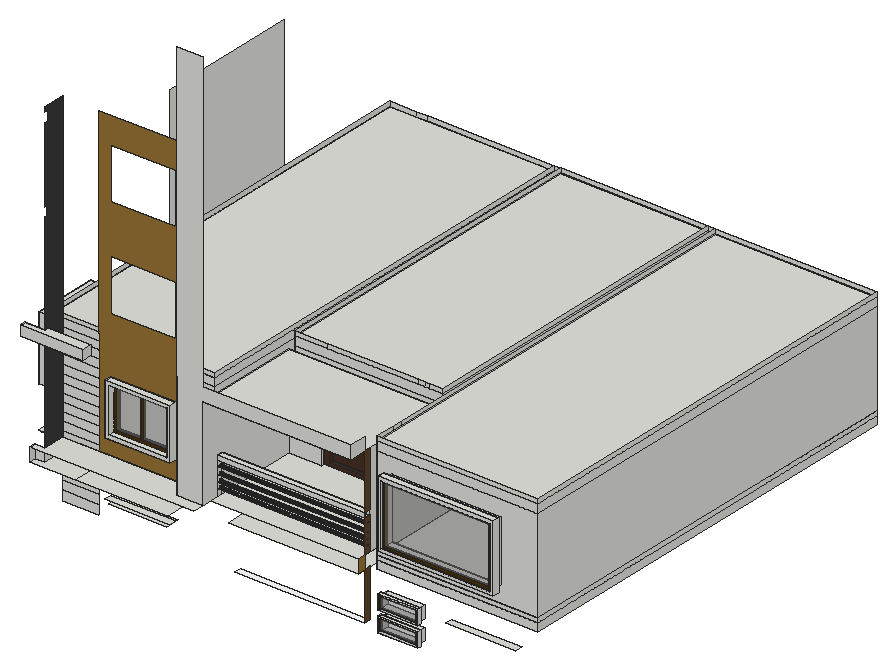
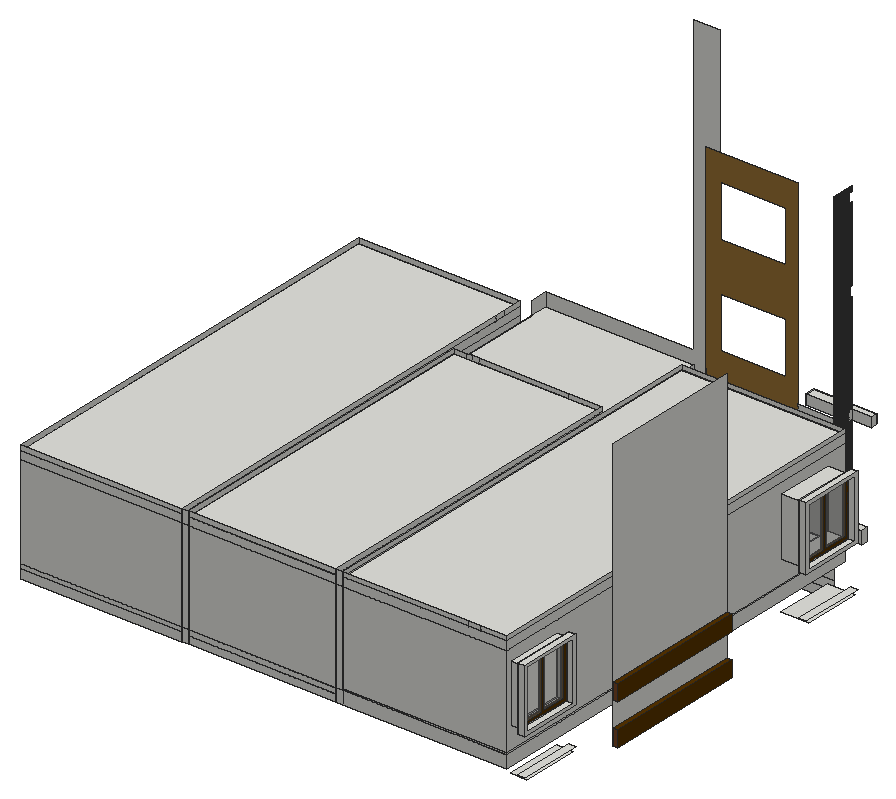
# SketchUp Ruby script. Lengths in inches.
U = 1.inch
M = Sketchup.active_model
def pt(a) = Geom::Point3d.new(a.map { |v| v * U })
def face(e, loops, mat)
  f = e.add_face(loops[0].map { |a| pt(a) })
  loops[1..].each { |l| e.add_face(l.map { |a| pt(a) }).erase! }
  f.material = f.back_material = mat if mat
  f
end
# faces: each face lists its corners as indices into pts; further lists are holes
def faces(e, pts, list, mat = nil) = list.each { |f| face(e, (f[0].is_a?(Array) ? f : [f]).map { |l| l.map { |i| pts[i] } }, mat) }
# xy, xz, yz: faces in a plane at the given z, y or x. An outline is a flat list of corners, or four numbers for a rectangle; further outlines are holes
def ring(l) = l.size == 4 ? [[l[0], l[1]], [l[2], l[1]], [l[2], l[3]], [l[0], l[3]]] : l.each_slice(2).to_a
def flat(e, list, mat, &to3) = list.each { |f| face(e, (f[0].is_a?(Array) ? f : [f]).map { |l| ring(l).map { |u, v| to3.(u, v) } }, mat) }
def xy(e, z, list, mat = nil) = flat(e, list, mat) { |x, y| [x, y, z] }
def xz(e, y, list, mat = nil) = flat(e, list, mat) { |x, z| [x, y, z] }
def yz(e, x, list, mat = nil) = flat(e, list, mat) { |y, z| [x, y, z] }
def lines(e, pts, list) = list.each { |a, b| e.add_line(pt(pts[a]), pt(pts[b])) }
# prism: a flat outline (further loops are holes) pulled along v
def prism(e, loops, v, mat = nil)
  f = face(e, loops, mat); d = Geom::Vector3d.new(v.map { |x| x * U })
  f.pushpull(f.normal.samedirection?(d) ? d.length : -d.length)
end
def box(e, o, s, mat = nil) = prism(e, [[o, [o[0] + s[0], o[1], o[2]], [o[0] + s[0], o[1] + s[1], o[2]], [o[0], o[1] + s[1], o[2]]]], [0, 0, s[2]], mat)
def at(x, y, z, deg = 0) = Geom::Transformation.translation(pt([x, y, z])) * Geom::Transformation.rotation(ORIGIN, Z_AXIS, deg.degrees)
def axes(o, x, y, z) = Geom::Transformation.new([*x, 0, *y, 0, *z, 0, *pt(o).to_a, 1])
def part(name) = M.definitions.add(name)
# library, detail: a bought-in or finely detailed component or shape, given as its bounding box
def library(name, o, s) = part(name).tap { |d| box(d.entities, o, s) }
def detail(e, o, s) = box(e.add_group.entities, o, s)
def put(e, d, t, mat = nil) = e.add_instance(d, t).tap { |i| i.material = mat if mat }
def group(e, t, mat = nil) = e.add_group.tap { |g| g.transformation = t; g.material = mat if mat }.entities
root = M.entities
M.materials.add("[Color C08]").color = [85, 51, 0]
M.materials.add("[Color D07]").color = [153, 114, 54]
M.materials.add("[Color D08]").color = [95, 67, 39]
M.materials.add("[Color M00]").color = [255, 255, 255]
M.materials.add("[Color M07]").color = [58, 58, 58]
M.materials.add("[Translucent Glass Gray]").color = [128, 128, 128]
M.materials["[Translucent Glass Gray]"].alpha = 0.5
M.materials.add("[Wood Veneer 01]").color = [71, 47, 37]
M.materials.add("[Wood Veneer 01]1").color = [120, 70, 37]
c1 = part("Group\#3")
xy(c1.entities,0,[[0,0,69.125,3.25]],"[Color C08]")
xy(c1.entities,1.72,[[1.72,0,67.41,3.25]],"[Color C08]")
xy(c1.entities,48.28,[[1.72,0,67.41,3.25]],"[Color C08]")
xy(c1.entities,50,[[0,0,69.125,3.25]],"[Color C08]")
xz(c1.entities,0,[[[0,0,69.125,50],[1.72,1.72,67.41,48.28]]],"[Color C08]")
xz(c1.entities,0,[[1.72,1.72,67.41,48.28]],"[Translucent Glass Gray]")
xz(c1.entities,3.25,[[[0,0,69.125,50],[1.72,1.72,67.41,48.28]]],"[Color C08]")
yz(c1.entities,0,[[0,0,3.25,50]],"[Color C08]")
yz(c1.entities,1.72,[[0,1.72,3.25,48.28]],"[Color C08]")
yz(c1.entities,67.41,[[0,1.72,3.25,48.28]],"[Color C08]")
yz(c1.entities,69.125,[[0,0,3.25,50]],"[Color C08]")
c2 = part("Group\#2")
xy(c2.entities,0,[[0,0,105.3125,8.625]],"[Wood Veneer 01]")
xy(c2.entities,6.5,[[6.5,0,98.81,8.625]],"[Wood Veneer 01]")
xy(c2.entities,132.37,[[6.5,0,98.81,8.625]],"[Wood Veneer 01]")
xy(c2.entities,138.875,[[0,0,105.3125,8.625]],"[Wood Veneer 01]")
xz(c2.entities,0,[[[0,0,105.3125,138.875],[6.5,6.5,98.81,132.37]]],"[Wood Veneer 01]")
xz(c2.entities,8.625,[[[0,0,105.3125,138.875],[6.5,6.5,98.81,132.37]],[6.5,6.5,98.81,132.37]],"[Wood Veneer 01]")
yz(c2.entities,0,[[0,0,8.625,138.875]],"[Wood Veneer 01]")
yz(c2.entities,6.5,[[0,6.5,8.625,132.37]],"[Wood Veneer 01]")
yz(c2.entities,98.81,[[0,6.5,8.625,132.37]],"[Wood Veneer 01]")
yz(c2.entities,105.3125,[[0,0,8.625,138.875]],"[Wood Veneer 01]")
c3 = part("Group\#4")
xy(c3.entities,0,[[0,0,0.4375,8.25]],"[Color C08]")
xy(c3.entities,9.875,[[0,0,0.4375,8.25]],"[Color C08]")
xz(c3.entities,0,[[0,0,0.4375,9.875]],"[Color C08]")
xz(c3.entities,0.45,[[0,0.45,0.4375,9.42]],"[Color C08]")
xz(c3.entities,4.05,[[0,0.49,0.4375,9.45]],"[Color C08]")
xz(c3.entities,4.38,[[0,0.49,0.4375,9.45]],"[Color C08]")
xz(c3.entities,7.8,[[0,0.45,0.4375,9.42]],"[Color C08]")
xz(c3.entities,8.25,[[0,0,0.4375,9.875]],"[Color C08]")
yz(c3.entities,0,[[[0,0,8.25,9.875],[0.45,0.45,4.05,0.49,4.05,9.45,0.45,9.42],[7.8,0.45,7.8,9.42,4.38,9.45,4.38,0.49]]],"[Color C08]")
yz(c3.entities,0,[[0.45,0.45,0.45,9.42,4.05,9.45,4.05,0.49],[7.8,0.45,4.38,0.49,4.38,9.45,7.8,9.42]],"[Translucent Glass Gray]")
yz(c3.entities,0.4375,[[[0,0,8.25,9.875],[0.45,0.45,0.45,9.42,4.05,9.45,4.05,0.49],[7.8,0.45,4.38,0.49,4.38,9.45,7.8,9.42]]],"[Color C08]")
p = [[0,4.05,0.49],[0,0.45,0.45],[0.4375,0.45,0.45],[0.4375,4.05,0.49],[0,7.8,0.45],[0,4.38,0.49],
  [0.4375,4.38,0.49],[0.4375,7.8,0.45],[0,0.45,9.42],[0,4.05,9.45],[0.4375,4.05,9.45],[0.4375,0.45,9.42],
  [0,4.38,9.45],[0,7.8,9.42],[0.4375,7.8,9.42],[0.4375,4.38,9.45]]
faces(c3.entities,p,[[0,1,2,3],[4,5,6,7],[8,9,10,11],[12,13,14,15]],"[Color C08]")
xy(root,214.49,[[507.06,205.375,558.75,209.375]])
xy(root,216.375,[[318.6875,209.375,486.25,218.375]],"[Color M00]")
xy(root,216.49,[[509.06,205.375,556.75,209.375],[509.06,209.375,556.75,218.375]])
xy(root,231.74,[[509.06,205.375,556.75,209.375],[509.06,209.375,556.75,218.375]])
xy(root,233.74,[[507.06,205.375,558.75,209.375]])
xy(root,240.37,[[507.06,205.375,558.75,209.375]])
xy(root,240.56,[[56.4375,423.72,63,608.17]],"[Color C08]")
xy(root,242.37,[[509.06,205.375,556.75,209.375],[509.06,209.375,556.75,218.375]])
xy(root,244.34,[[162.4,200.375,237.77,209.375],[162.4,209.375,237.77,218.375]])
xy(root,248.34,[[158.4,200.375,241.77,209.375]])
xy(root,253.18,[[591.14,209.375,681.47,218.375]])
xy(root,256.3125,[[337.77,326.375,453.52,335.375]])
xy(root,257.62,[[509.06,205.375,556.75,209.375],[509.06,209.375,556.75,218.375]])
xy(root,259.62,[[507.06,205.375,558.75,209.375]])
xy(root,261.95,[[56.4375,423.72,63,608.17]],"[Color C08]")
xy(root,264.95,[[39.625,245.8125,48.625,321.0625],[48.625,245.8125,75,321.0625]])
xy(root,268.95,[[39.625,241.8125,48.625,325.0625]])
xy(root,270.1,[[54,683.03,63,757.4],[63,683.03,75,757.4]])
xy(root,274.1,[[54,679.03,63,761.4]])
xy(root,278,[[83.63,172.6875,83.63,180.75,95.94,180.75,95.94,209.375,143.14,209.375,143.14,172.6875],[143.14,172.6875,261.34,209.375],[318.6875,199.5625,318.6875,227.625,295.1875,227.625,295.1875,326.375,486.25,326.375,486.25,199.5625]])
xy(root,287.9375,[[295.1875,335.375,486.25,764.25]])
xy(root,289,[[495.25,218.375,703.3125,764.25]])
xy(root,293.62,[[56.4375,423.72,63,608.17]],"[Color C08]")
xy(root,295,[[83.63,172.6875,295.1875,172.6875,295.1875,187.375,261.34,187.375,261.34,209.375,95.94,209.375,95.94,180.75,83.63,180.75],[295.1875,199.5625,486.25,199.5625,486.25,326.375,453.52,326.375,453.52,335.375,337.77,335.375,337.77,326.375,295.1875,326.375],[75,218.375,286.1875,764.25],[495.25,218.375,703.3125,764.25],[295.1875,335.375,486.25,764.25]])
xy(root,296.3125,[[75,218.375,286.1875,764.25]])
xy(root,312.03,[[510.53,200.375,659.59,209.375]])
xy(root,315.01,[[56.4375,423.72,63,608.17]],"[Color C08]")
xy(root,316.03,[[514.53,200.375,655.59,209.375],[514.53,209.375,655.59,218.375]])
xy(root,319.84,[[158.4,200.375,241.77,209.375]])
xy(root,321.73,[[54,679.03,63,761.4]])
xy(root,322.38,[[39.625,241.8125,48.625,325.0625]])
xy(root,323.84,[[162.4,200.375,237.77,209.375],[162.4,209.375,237.77,218.375]])
xy(root,325.73,[[54,683.03,63,757.4],[63,683.03,75,757.4]])
xy(root,326.38,[[39.625,245.8125,48.625,321.0625],[48.625,245.8125,75,321.0625]])
xy(root,337.37,[[295.1875,210,486.25,218.375]])
xy(root,343,[[295.1875,210,486.25,218.375]])
xy(root,382.03,[[162.4,200.375,237.77,209.375],[162.4,209.375,237.77,218.375]])
xy(root,386.03,[[158.4,200.375,241.77,209.375]])
xy(root,393.3125,[[337.77,326.375,453.52,335.375]])
xy(root,394.84,[[514.53,200.375,655.59,209.375],[514.53,209.375,655.59,218.375]])
xy(root,398.84,[[510.53,200.375,659.59,209.375]])
xy(root,400.1,[[54,683.03,63,757.4],[63,683.03,75,757.4]])
xy(root,401.63,[[39.625,245.8125,48.625,321.0625],[48.625,245.8125,75,321.0625]])
xy(root,404.1,[[54,679.03,63,761.4]])
xy(root,405.63,[[39.625,241.8125,48.625,325.0625]])
xy(root,415,[[295.1875,187.375,486.25,326.375]])
xy(root,418.67,[[70.87,172.6875,70.87,180.75,95.94,180.75,95.94,186.375,151.38,186.375,151.38,172.6875]])
xy(root,426,[[75,218.375,286.1875,764.25],[495.25,218.375,703.3125,764.25],[295.1875,335.375,486.25,764.25]])
xy(root,431.12,[[70.87,172.6875,151.38,172.6875,151.38,186.375,95.94,186.375,95.94,180.75,70.87,180.75]])
xz(root,172.6875,[[70.87,418.67,151.38,431.12]])
xz(root,180.75,[[83.63,278,95.94,295],[70.87,418.67,95.94,431.12]])
xz(root,186.375,[[95.94,418.67,151.38,431.12]])
xz(root,187.375,[[261.34,295,295.1875,295,295.1875,415,486.25,415,486.25,432,295.1875,432,295.1875,814.1875,261.34,814.1875]])
xz(root,200.375,[[[510.53,312.03,659.59,398.84],[514.53,316.03,655.59,394.84]],[[158.4,319.84,241.77,386.03],[162.4,323.84,237.77,382.03]]])
xz(root,205.375,[[[507.06,214.49,558.75,233.74],[509.06,216.49,556.75,231.74]],[[507.06,240.37,558.75,259.62],[509.06,242.37,556.75,257.62]]])
xz(root,209.375,[[[507.06,214.49,558.75,233.74],[509.06,216.49,556.75,231.74]],[95.94,220.9,143.14,233.09],[95.94,233.09,143.14,245.27],[[507.06,240.37,558.75,259.62],[509.06,242.37,556.75,257.62]],[95.94,245.27,143.14,257.46],
  [95.94,257.46,143.14,268.52],[95.94,268.52,143.14,278],[95.94,278,261.34,295],[95.94,295,143.14,301.71],[95.94,301.71,143.14,312.77],
  [[510.53,312.03,659.59,398.84],[514.53,316.03,655.59,394.84]],[95.94,312.77,143.14,323.84],[[158.4,319.84,241.77,386.03],[162.4,323.84,237.77,382.03]],[95.94,323.84,143.14,334.9],[95.94,334.9,143.14,345.96],
  [95.94,345.96,143.14,357.02],[95.94,357.02,143.14,368.09],[95.94,368.09,143.14,379.15],[95.94,379.15,143.14,390.21],[95.94,390.21,143.14,401.27],
  [95.94,401.27,143.14,412.34],[95.94,412.34,143.14,422.52],[95.94,422.52,143.14,432.71]])
xz(root,209.375,[[[143.14,295,261.34,689],[158.4,319.84,241.77,386.03],[158.4,459.4,241.77,525.59],[158.4,588.78,241.77,654.97]]],"[Color D07]")
xz(root,210,[[295.1875,337.37,486.25,343]])
xz(root,218.375,[[495.25,278,703.3125,289],[495.25,289,703.3125,295],[75,295,286.1875,296.3125],[[495.25,295,703.3125,415],[514.53,316.03,655.59,394.84]],[[75,296.3125,286.1875,415],[162.4,323.84,237.77,382.03]],
  [295.1875,337.37,486.25,343],[75,415,286.1875,426],[495.25,415,703.3125,426],[75,426,286.1875,432],[495.25,426,703.3125,432]])
xz(root,241.8125,[[39.625,322.38,48.625,405.63]])
xz(root,245.8125,[[39.625,326.38,48.625,401.63],[48.625,326.38,75,401.63]])
xz(root,321.0625,[[39.625,326.38,48.625,401.63],[48.625,326.38,75,401.63]])
xz(root,325.0625,[[39.625,322.38,48.625,405.63]])
xz(root,326.375,[[295.1875,295,337.77,295,337.77,393.3125,453.52,393.3125,453.52,295,486.25,295,486.25,415,295.1875,415]])
xz(root,335.375,[[295.1875,278,486.25,287.9375],[295.1875,287.9375,326.15,295],[326.15,287.9375,337.77,295],[337.77,287.9375,453.52,295],[453.52,287.9375,486.25,295],
  [295.1875,295,295.1875,415,486.25,415,486.25,295,453.52,295,453.52,393.3125,337.77,393.3125,337.77,295],[295.1875,415,486.25,426],[295.1875,426,338.07,432],[338.07,426,453.82,432],[453.82,426,463.6,432],
  [463.6,426,470.04,432],[470.04,426,486.25,432]])
xz(root,423.72,[[56.4375,240.56,63,261.95],[56.4375,293.62,63,315.01]],"[Wood Veneer 01]1")
xz(root,608.17,[[56.4375,240.56,63,261.95],[56.4375,293.62,63,315.01]],"[Wood Veneer 01]1")
xz(root,679.03,[[54,321.73,63,404.1]])
xz(root,683.03,[[54,325.73,63,400.1],[63,325.73,75,400.1]])
xz(root,757.4,[[54,325.73,63,400.1],[63,325.73,75,400.1]])
xz(root,761.4,[[54,321.73,63,404.1]])
xz(root,764.25,[[75,278,286.1875,295],[286.1875,278,295.1875,295],[295.1875,278,486.25,287.9375],[486.25,278,495.25,295],[495.25,278,703.3125,289],
  [295.1875,287.9375,486.25,295],[495.25,289,703.3125,295],[75,295,286.1875,296.3125],[286.1875,295,295.1875,415],[295.1875,295,486.25,415],
  [486.25,295,495.25,415],[495.25,295,703.3125,415],[75,296.3125,286.1875,415],[75,415,286.1875,426],[286.1875,415,295.1875,432],
  [295.1875,415,486.25,426],[486.25,415,495.25,432],[495.25,415,703.3125,426],[75,426,108.93,432],[108.93,426,123.62,432],
  [123.62,426,286.1875,432],[295.1875,426,486.25,432],[495.25,426,703.3125,432]])
yz(root,39.625,[[[241.8125,322.38,325.0625,405.63],[245.8125,326.38,321.0625,401.63]]])
yz(root,48.625,[[[241.8125,322.38,325.0625,405.63],[245.8125,326.38,321.0625,401.63]]])
yz(root,54,[[[679.03,321.73,761.4,404.1],[683.03,325.73,757.4,400.1]]])
yz(root,56.4375,[[423.72,240.56,608.17,261.95],[423.72,293.62,608.17,315.01]],"[Color C08]")
yz(root,63,[[423.72,261.95,608.17,293.62],[423.72,315.01,608.17,590.06],[[679.03,321.73,761.4,404.1],[683.03,325.73,757.4,400.1]]])
yz(root,63,[[423.72,240.56,608.17,261.95],[423.72,293.62,608.17,315.01]],"[Wood Veneer 01]1")
yz(root,70.87,[[172.6875,418.67,180.75,431.12]])
yz(root,75,[[218.375,278,764.25,295],[218.375,295,764.25,296.3125],[[218.375,296.3125,764.25,415],[245.8125,326.38,321.0625,401.63],[683.03,325.73,757.4,400.1]],[218.375,415,764.25,426],[218.375,426,764.25,432]])
yz(root,83.63,[[172.6875,278,180.75,295]])
yz(root,95.94,[[180.75,278,209.375,295],[180.75,418.67,186.375,431.12]])
yz(root,95.94,[[180.75,295,209.375,295,209.375,689,180.75,689,180.75,682.81,185.5,682.81,185.5,670.36,180.75,670.36,180.75,573.81,184.6875,573.81,184.6875,561.36,180.75,561.36,180.75,431.12,186.375,431.12,186.375,418.67,180.75,418.67]],"[Color M07]")
yz(root,151.38,[[172.6875,418.67,186.375,431.12]])
yz(root,158.4,[[200.375,319.84,209.375,386.03]])
yz(root,162.4,[[200.375,323.84,209.375,382.03],[209.375,323.84,218.375,382.03]])
yz(root,237.77,[[200.375,323.84,209.375,382.03],[209.375,323.84,218.375,382.03]])
yz(root,241.77,[[200.375,319.84,209.375,386.03]])
yz(root,261.34,[[187.375,295,209.375,415],[187.375,415,209.375,432]])
yz(root,286.1875,[[218.375,295,764.25,296.3125],[218.375,296.3125,764.25,415],[218.375,415,764.25,426],[218.375,426,764.25,432]])
yz(root,295.1875,[[335.375,278,764.25,287.9375],[335.375,287.9375,764.25,295],[187.375,295,210,295,210,343,218.375,343,218.375,295,326.375,295,326.375,415,187.375,415],[[210,295,218.375,337.37],[214.19,302.13,213.74,302.19,213.32,302.37,212.96,302.65,212.68,303.01,212.5,303.43,212.44,303.88,212.5,304.34,212.68,304.76,212.96,305.12,213.32,305.4,213.74,305.57,214.19,305.63,214.65,305.57,215.07,305.4,215.43,305.12,215.71,304.76,215.88,304.34,215.94,303.88,215.88,303.43,215.71,303.01,215.43,302.65,215.07,302.37,214.65,302.19],[214.19,309.82,213.74,309.88,213.32,310.06,212.96,310.33,212.68,310.7,212.5,311.12,212.44,311.57,212.5,312.02,212.68,312.45,212.96,312.81,213.32,313.09,213.74,313.26,214.19,313.32,214.65,313.26,215.07,313.09,215.43,312.81,215.71,312.45,215.88,312.02,215.94,311.57,215.88,311.12,215.71,310.7,215.43,310.33,215.07,310.06,214.65,309.88],[214.19,318.2,213.74,318.26,213.32,318.43,212.96,318.71,212.68,319.07,212.5,319.49,212.44,319.95,212.5,320.4,212.68,320.82,212.96,321.18,213.32,321.46,213.74,321.64,214.19,321.7,214.65,321.64,215.07,321.46,215.43,321.18,215.71,320.82,215.88,320.4,215.94,319.95,215.88,319.49,215.71,319.07,215.43,318.71,215.07,318.43,214.65,318.26],[214.19,327.95,213.74,328.01,213.32,328.18,212.96,328.46,212.68,328.82,212.5,329.24,212.44,329.7,212.5,330.15,212.68,330.57,212.96,330.93,213.32,331.21,213.74,331.39,214.19,331.45,214.65,331.39,215.07,331.21,215.43,330.93,215.71,330.57,215.88,330.15,215.94,329.7,215.88,329.24,215.71,328.82,215.43,328.46,215.07,328.18,214.65,328.01]],[335.375,295,764.25,415],
  [214.19,302.13,213.74,302.19,213.32,302.37,212.96,302.65,212.68,303.01,212.5,303.43,212.44,303.88,212.5,304.34,212.68,304.76,212.96,305.12,213.32,305.4,213.74,305.57,214.19,305.63,214.65,305.57,215.07,305.4,215.43,305.12,215.71,304.76,215.88,304.34,215.94,303.88,215.88,303.43,215.71,303.01,215.43,302.65,215.07,302.37,214.65,302.19],[214.19,309.82,213.74,309.88,213.32,310.06,212.96,310.33,212.68,310.7,212.5,311.12,212.44,311.57,212.5,312.02,212.68,312.45,212.96,312.81,213.32,313.09,213.74,313.26,214.19,313.32,214.65,313.26,215.07,313.09,215.43,312.81,215.71,312.45,215.88,312.02,215.94,311.57,215.88,311.12,215.71,310.7,215.43,310.33,215.07,310.06,214.65,309.88],[214.19,318.2,213.74,318.26,213.32,318.43,212.96,318.71,212.68,319.07,212.5,319.49,212.44,319.95,212.5,320.4,212.68,320.82,212.96,321.18,213.32,321.46,213.74,321.64,214.19,321.7,214.65,321.64,215.07,321.46,215.43,321.18,215.71,320.82,215.88,320.4,215.94,319.95,215.88,319.49,215.71,319.07,215.43,318.71,215.07,318.43,214.65,318.26],[214.19,327.95,213.74,328.01,213.32,328.18,212.96,328.46,212.68,328.82,212.5,329.24,212.44,329.7,212.5,330.15,212.68,330.57,212.96,330.93,213.32,331.21,213.74,331.39,214.19,331.45,214.65,331.39,215.07,331.21,215.43,330.93,215.71,330.57,215.88,330.15,215.94,329.7,215.88,329.24,215.71,328.82,215.43,328.46,215.07,328.18,214.65,328.01],[210,337.37,218.375,343],
  [335.375,415,764.25,426],[335.375,426,764.25,432]])
yz(root,337.77,[[326.375,295,335.375,393.3125]])
yz(root,453.52,[[326.375,295,335.375,393.3125]])
yz(root,486.25,[[335.375,278,764.25,287.9375],[335.375,287.9375,764.25,295],[218.375,295,326.375,415],[335.375,295,764.25,415],[187.375,415,209.375,432],
  [335.375,415,764.25,426],[335.375,426,764.25,432]])
yz(root,486.25,[[199.5625,278,209.375,295]],"[Color D07]")
yz(root,486.25,[[209.375,216.375,218.375,278],[[209.375,295,209.375,415,218.375,415,218.375,343,210,343,210,337.37,218.375,337.37,218.375,295],[214.19,327.95,214.65,328.01,215.07,328.18,215.43,328.46,215.71,328.82,215.88,329.24,215.94,329.7,215.88,330.15,215.71,330.57,215.43,330.93,215.07,331.21,214.65,331.39,214.19,331.45,213.74,331.39,213.32,331.21,212.96,330.93,212.68,330.57,212.5,330.15,212.44,329.7,212.5,329.24,212.68,328.82,212.96,328.46,213.32,328.18,213.74,328.01],[214.19,318.2,214.65,318.26,215.07,318.43,215.43,318.71,215.71,319.07,215.88,319.49,215.94,319.95,215.88,320.4,215.71,320.82,215.43,321.18,215.07,321.46,214.65,321.64,214.19,321.7,213.74,321.64,213.32,321.46,212.96,321.18,212.68,320.82,212.5,320.4,212.44,319.95,212.5,319.49,212.68,319.07,212.96,318.71,213.32,318.43,213.74,318.26],[214.19,309.82,214.65,309.88,215.07,310.06,215.43,310.33,215.71,310.7,215.88,311.12,215.94,311.57,215.88,312.02,215.71,312.45,215.43,312.81,215.07,313.09,214.65,313.26,214.19,313.32,213.74,313.26,213.32,313.09,212.96,312.81,212.68,312.45,212.5,312.02,212.44,311.57,212.5,311.12,212.68,310.7,212.96,310.33,213.32,310.06,213.74,309.88],[214.19,302.13,214.65,302.19,215.07,302.37,215.43,302.65,215.71,303.01,215.88,303.43,215.94,303.88,215.88,304.34,215.71,304.76,215.43,305.12,215.07,305.4,214.65,305.57,214.19,305.63,213.74,305.57,213.32,305.4,212.96,305.12,212.68,304.76,212.5,304.34,212.44,303.88,212.5,303.43,212.68,303.01,212.96,302.65,213.32,302.37,213.74,302.19]]],"[Color D08]")
yz(root,495.25,[[218.375,278,764.25,289],[218.375,289,226.47,295],[226.47,289,235.53,295],[235.53,289,764.25,295],[218.375,295,764.25,415],
  [218.375,415,764.25,426],[218.375,426,243.49,432],[243.49,426,256.74,432],[256.74,426,764.25,432]])
yz(root,507.06,[[205.375,214.49,209.375,233.74],[205.375,240.37,209.375,259.62]])
yz(root,509.06,[[205.375,216.49,209.375,231.74],[209.375,216.49,218.375,231.74],[205.375,242.37,209.375,257.62],[209.375,242.37,218.375,257.62]])
yz(root,510.53,[[200.375,312.03,209.375,398.84]])
yz(root,514.53,[[200.375,316.03,209.375,394.84],[209.375,316.03,218.375,394.84]])
yz(root,556.75,[[205.375,216.49,209.375,231.74],[209.375,216.49,218.375,231.74],[205.375,242.37,209.375,257.62],[209.375,242.37,218.375,257.62]])
yz(root,558.75,[[205.375,214.49,209.375,233.74],[205.375,240.37,209.375,259.62]])
yz(root,655.59,[[200.375,316.03,209.375,394.84],[209.375,316.03,218.375,394.84]])
yz(root,659.59,[[200.375,312.03,209.375,398.84]])
yz(root,703.3125,[[218.375,278,764.25,289],[218.375,289,764.25,295],[218.375,295,764.25,415],[218.375,415,764.25,426],[218.375,426,764.25,432]])
p = [[295.1875,213.74,302.19],[295.1875,214.19,302.13],[486.25,214.19,302.13],[486.25,213.74,302.19],[295.1875,214.65,302.19],[486.25,214.65,302.19],
  [295.1875,213.32,302.37],[486.25,213.32,302.37],[295.1875,215.07,302.37],[486.25,215.07,302.37],[295.1875,212.96,302.65],[486.25,212.96,302.65],
  [295.1875,215.43,302.65],[486.25,215.43,302.65],[295.1875,212.68,303.01],[486.25,212.68,303.01],[295.1875,215.71,303.01],[486.25,215.71,303.01],
  [295.1875,212.5,303.43],[486.25,212.5,303.43],[295.1875,215.88,303.43],[486.25,215.88,303.43],[295.1875,212.44,303.88],[486.25,212.44,303.88],
  [295.1875,215.94,303.88],[486.25,215.94,303.88],[295.1875,212.5,304.34],[486.25,212.5,304.34],[295.1875,215.88,304.34],[486.25,215.88,304.34],
  [295.1875,212.68,304.76],[486.25,212.68,304.76],[295.1875,215.71,304.76],[486.25,215.71,304.76],[295.1875,212.96,305.12],[486.25,212.96,305.12],
  [295.1875,215.43,305.12],[486.25,215.43,305.12],[295.1875,213.32,305.4],[486.25,213.32,305.4],[295.1875,215.07,305.4],[486.25,215.07,305.4],
  [295.1875,213.74,305.57],[486.25,213.74,305.57],[295.1875,214.65,305.57],[486.25,214.65,305.57],[295.1875,214.19,305.63],[486.25,214.19,305.63],
  [295.1875,213.74,309.88],[295.1875,214.19,309.82],[486.25,214.19,309.82],[486.25,213.74,309.88],[295.1875,214.65,309.88],[486.25,214.65,309.88],
  [295.1875,213.32,310.06],[486.25,213.32,310.06],[295.1875,215.07,310.06],[486.25,215.07,310.06],[295.1875,212.96,310.33],[486.25,212.96,310.33],
  [295.1875,215.43,310.33],[486.25,215.43,310.33],[295.1875,212.68,310.7],[486.25,212.68,310.7],[295.1875,215.71,310.7],[486.25,215.71,310.7],
  [295.1875,212.5,311.12],[486.25,212.5,311.12],[295.1875,215.88,311.12],[486.25,215.88,311.12],[295.1875,212.44,311.57],[486.25,212.44,311.57],
  [295.1875,215.94,311.57],[486.25,215.94,311.57],[295.1875,212.5,312.02],[486.25,212.5,312.02],[295.1875,215.88,312.02],[486.25,215.88,312.02],
  [295.1875,212.68,312.45],[486.25,212.68,312.45],[295.1875,215.71,312.45],[486.25,215.71,312.45],[295.1875,212.96,312.81],[486.25,212.96,312.81],
  [295.1875,215.43,312.81],[486.25,215.43,312.81],[295.1875,213.32,313.09],[486.25,213.32,313.09],[295.1875,215.07,313.09],[486.25,215.07,313.09],
  [295.1875,213.74,313.26],[486.25,213.74,313.26],[295.1875,214.65,313.26],[486.25,214.65,313.26],[295.1875,214.19,313.32],[486.25,214.19,313.32],
  [295.1875,213.74,318.26],[295.1875,214.19,318.2],[486.25,214.19,318.2],[486.25,213.74,318.26],[295.1875,214.65,318.26],[486.25,214.65,318.26],
  [295.1875,213.32,318.43],[486.25,213.32,318.43],[295.1875,215.07,318.43],[486.25,215.07,318.43],[295.1875,212.96,318.71],[486.25,212.96,318.71],
  [295.1875,215.43,318.71],[486.25,215.43,318.71],[295.1875,212.68,319.07],[486.25,212.68,319.07],[295.1875,215.71,319.07],[486.25,215.71,319.07],
  [295.1875,212.5,319.49],[486.25,212.5,319.49],[295.1875,215.88,319.49],[486.25,215.88,319.49],[295.1875,212.44,319.95],[486.25,212.44,319.95],
  [295.1875,215.94,319.95],[486.25,215.94,319.95],[295.1875,212.5,320.4],[486.25,212.5,320.4],[295.1875,215.88,320.4],[486.25,215.88,320.4],
  [295.1875,212.68,320.82],[486.25,212.68,320.82],[295.1875,215.71,320.82],[486.25,215.71,320.82],[295.1875,212.96,321.18],[486.25,212.96,321.18],
  [295.1875,215.43,321.18],[486.25,215.43,321.18],[295.1875,213.32,321.46],[486.25,213.32,321.46],[295.1875,215.07,321.46],[486.25,215.07,321.46],
  [295.1875,213.74,321.64],[486.25,213.74,321.64],[295.1875,214.65,321.64],[486.25,214.65,321.64],[295.1875,214.19,321.7],[486.25,214.19,321.7],
  [295.1875,213.74,328.01],[295.1875,214.19,327.95],[486.25,214.19,327.95],[486.25,213.74,328.01],[295.1875,214.65,328.01],[486.25,214.65,328.01],
  [295.1875,213.32,328.18],[486.25,213.32,328.18],[295.1875,215.07,328.18],[486.25,215.07,328.18],[295.1875,212.96,328.46],[486.25,212.96,328.46],
  [295.1875,215.43,328.46],[486.25,215.43,328.46],[295.1875,212.68,328.82],[486.25,212.68,328.82],[295.1875,215.71,328.82],[486.25,215.71,328.82],
  [295.1875,212.5,329.24],[486.25,212.5,329.24],[295.1875,215.88,329.24],[486.25,215.88,329.24],[295.1875,212.44,329.7],[486.25,212.44,329.7],
  [295.1875,215.94,329.7],[486.25,215.94,329.7],[295.1875,212.5,330.15],[486.25,212.5,330.15],[295.1875,215.88,330.15],[486.25,215.88,330.15],
  [295.1875,212.68,330.57],[486.25,212.68,330.57],[295.1875,215.71,330.57],[486.25,215.71,330.57],[295.1875,212.96,330.93],[486.25,212.96,330.93],
  [295.1875,215.43,330.93],[486.25,215.43,330.93],[295.1875,213.32,331.21],[486.25,213.32,331.21],[295.1875,215.07,331.21],[486.25,215.07,331.21],
  [295.1875,213.74,331.39],[486.25,213.74,331.39],[295.1875,214.65,331.39],[486.25,214.65,331.39],[295.1875,214.19,331.45],[486.25,214.19,331.45],
  [95.94,209.375,290.65],[143.14,209.375,290.65],[95.94,209.375,279.59],[143.14,209.375,279.59]]
faces(root,p,[[0,1,2,3],[1,4,5,2],[6,0,3,7],[4,8,9,5],[10,6,7,11],[8,12,13,9],[14,10,11,15],[12,16,17,13],
  [18,14,15,19],[16,20,21,17],[22,18,19,23],[20,24,25,21],[26,22,23,27],[24,28,29,25],[30,26,27,31],[28,32,33,29],
  [34,30,31,35],[32,36,37,33],[38,34,35,39],[36,40,41,37],[42,38,39,43],[40,44,45,41],[46,42,43,47],[44,46,47,45],
  [48,49,50,51],[49,52,53,50],[54,48,51,55],[52,56,57,53],[58,54,55,59],[56,60,61,57],[62,58,59,63],[60,64,65,61],
  [66,62,63,67],[64,68,69,65],[70,66,67,71],[68,72,73,69],[74,70,71,75],[72,76,77,73],[78,74,75,79],[76,80,81,77],
  [82,78,79,83],[80,84,85,81],[86,82,83,87],[84,88,89,85],[90,86,87,91],[88,92,93,89],[94,90,91,95],[92,94,95,93],
  [96,97,98,99],[97,100,101,98],[102,96,99,103],[100,104,105,101],[106,102,103,107],[104,108,109,105],[110,106,107,111],[108,112,113,109],
  [114,110,111,115],[112,116,117,113],[118,114,115,119],[116,120,121,117],[122,118,119,123],[120,124,125,121],[126,122,123,127],[124,128,129,125],
  [130,126,127,131],[128,132,133,129],[134,130,131,135],[132,136,137,133],[138,134,135,139],[136,140,141,137],[142,138,139,143],[140,142,143,141],
  [144,145,146,147],[145,148,149,146],[150,144,147,151],[148,152,153,149],[154,150,151,155],[152,156,157,153],[158,154,155,159],[156,160,161,157],
  [162,158,159,163],[160,164,165,161],[166,162,163,167],[164,168,169,165],[170,166,167,171],[168,172,173,169],[174,170,171,175],[172,176,177,173],
  [178,174,175,179],[176,180,181,177],[182,178,179,183],[180,184,185,181],[186,182,183,187],[184,188,189,185],[190,186,187,191],[188,190,191,189]])
lines(root,p,[[192,193],[194,195]])
put(root,c1,axes([509.06,206,216.49],[0.68987,0,0],[0,0.35,0],[0,0,0.305]))
put(root,c1,axes([509.06,206,242.37],[0.68987,0,0],[0,0.35,0],[0,0,0.305]))
put(root,c2,axes([337.77,329.83,295],[1.09911,0,0],[0,0.6,0],[0,0,0.70792]))
put(root,c1,axes([514.53,202.875,316.03],[2.04069,0,0],[0,1,0],[0,0,1.57625]))
put(root,c3,axes([237.77,209.375,323.84],[0,6.04632,0],[-9.13636,0,0],[0,0,5.89241]))
put(root,c3,axes([63,683.03,325.73],[8.6376,0,0],[0,9.01515,0],[0,0,7.53165]))
put(root,c3,axes([48.625,245.8125,326.38],[8.6376,0,0],[0,9.1053,0],[0,0,7.62025]))
